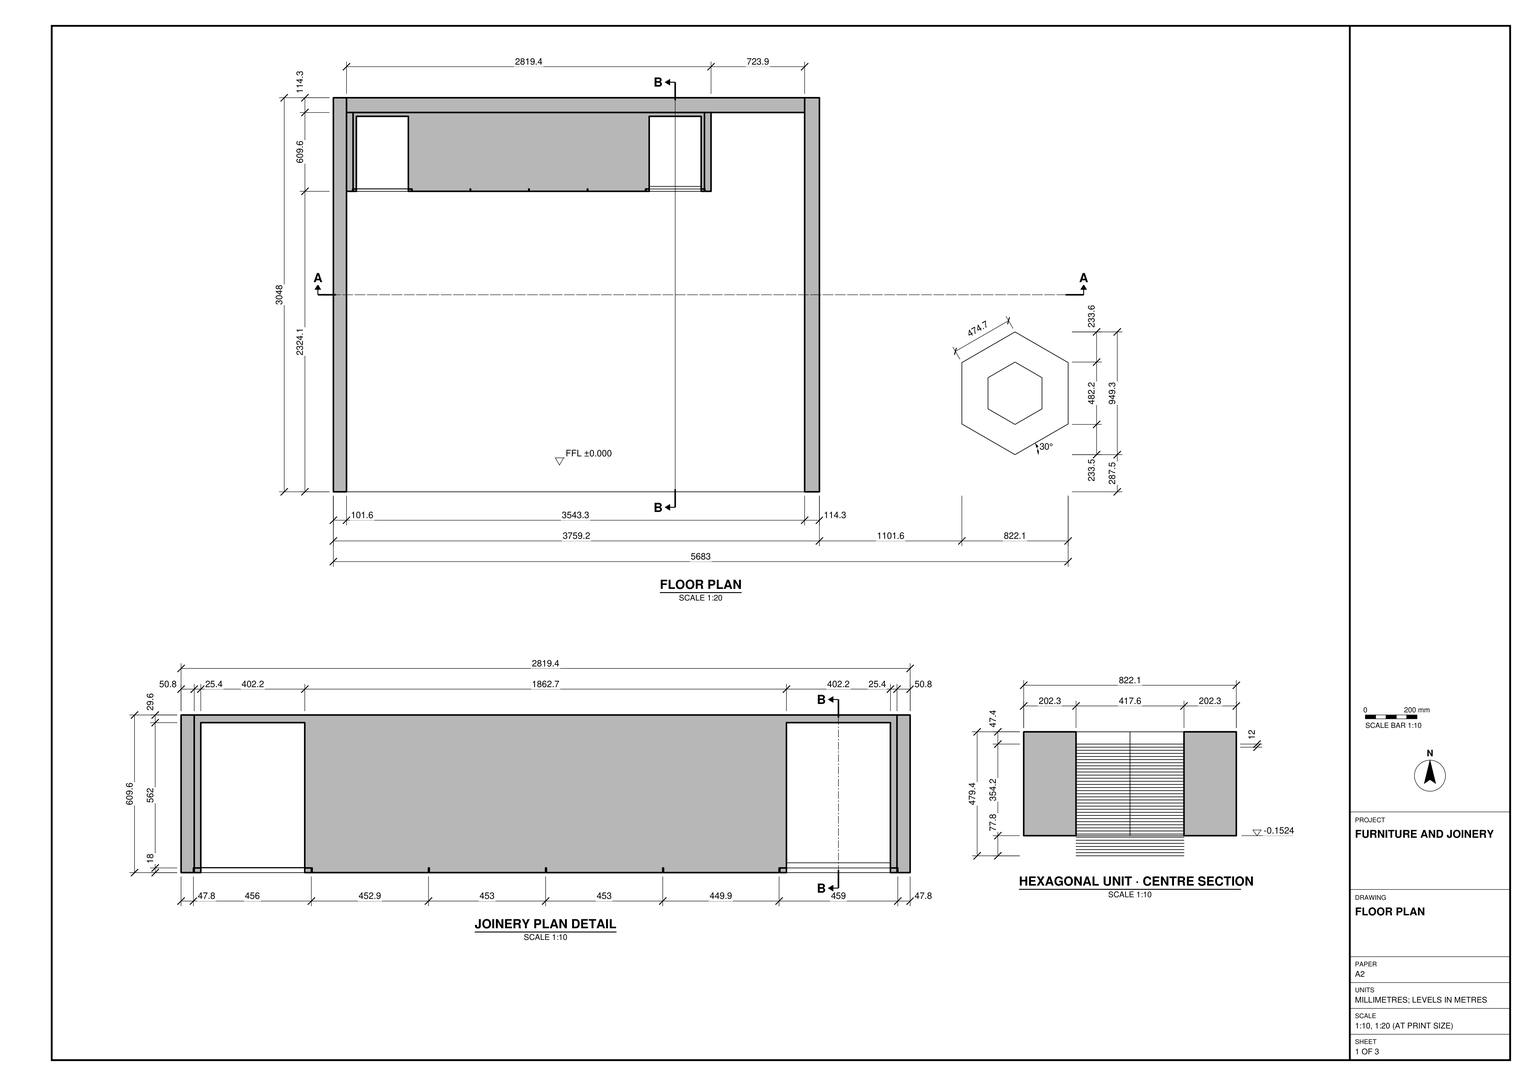
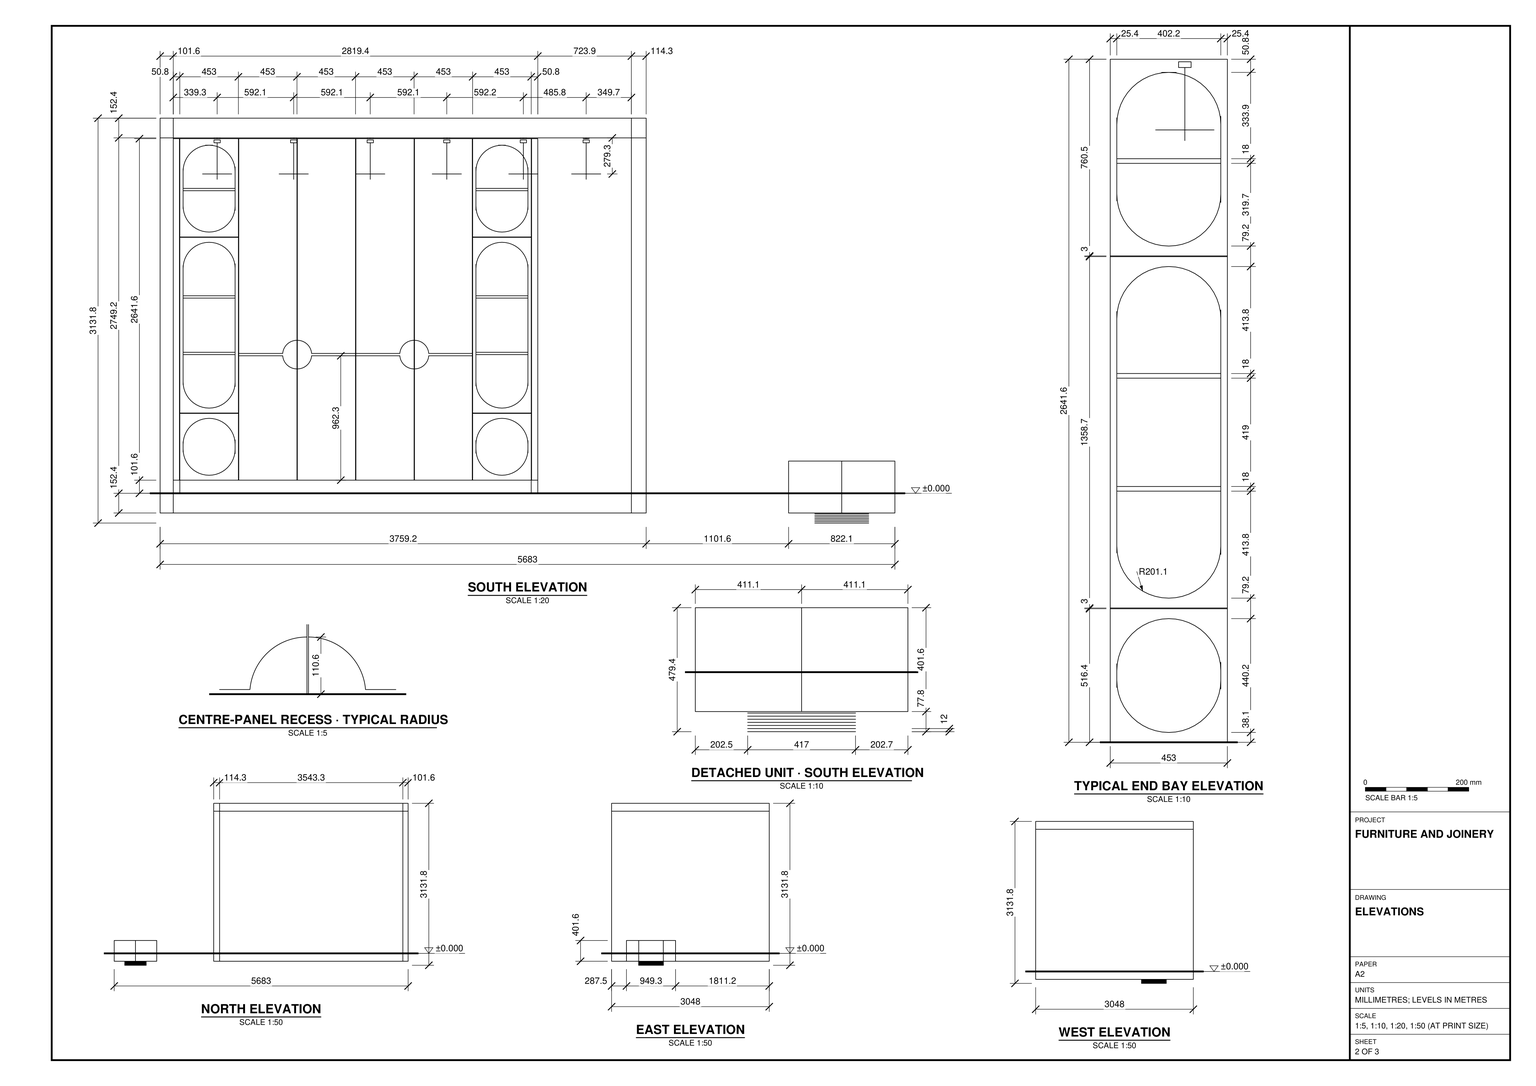
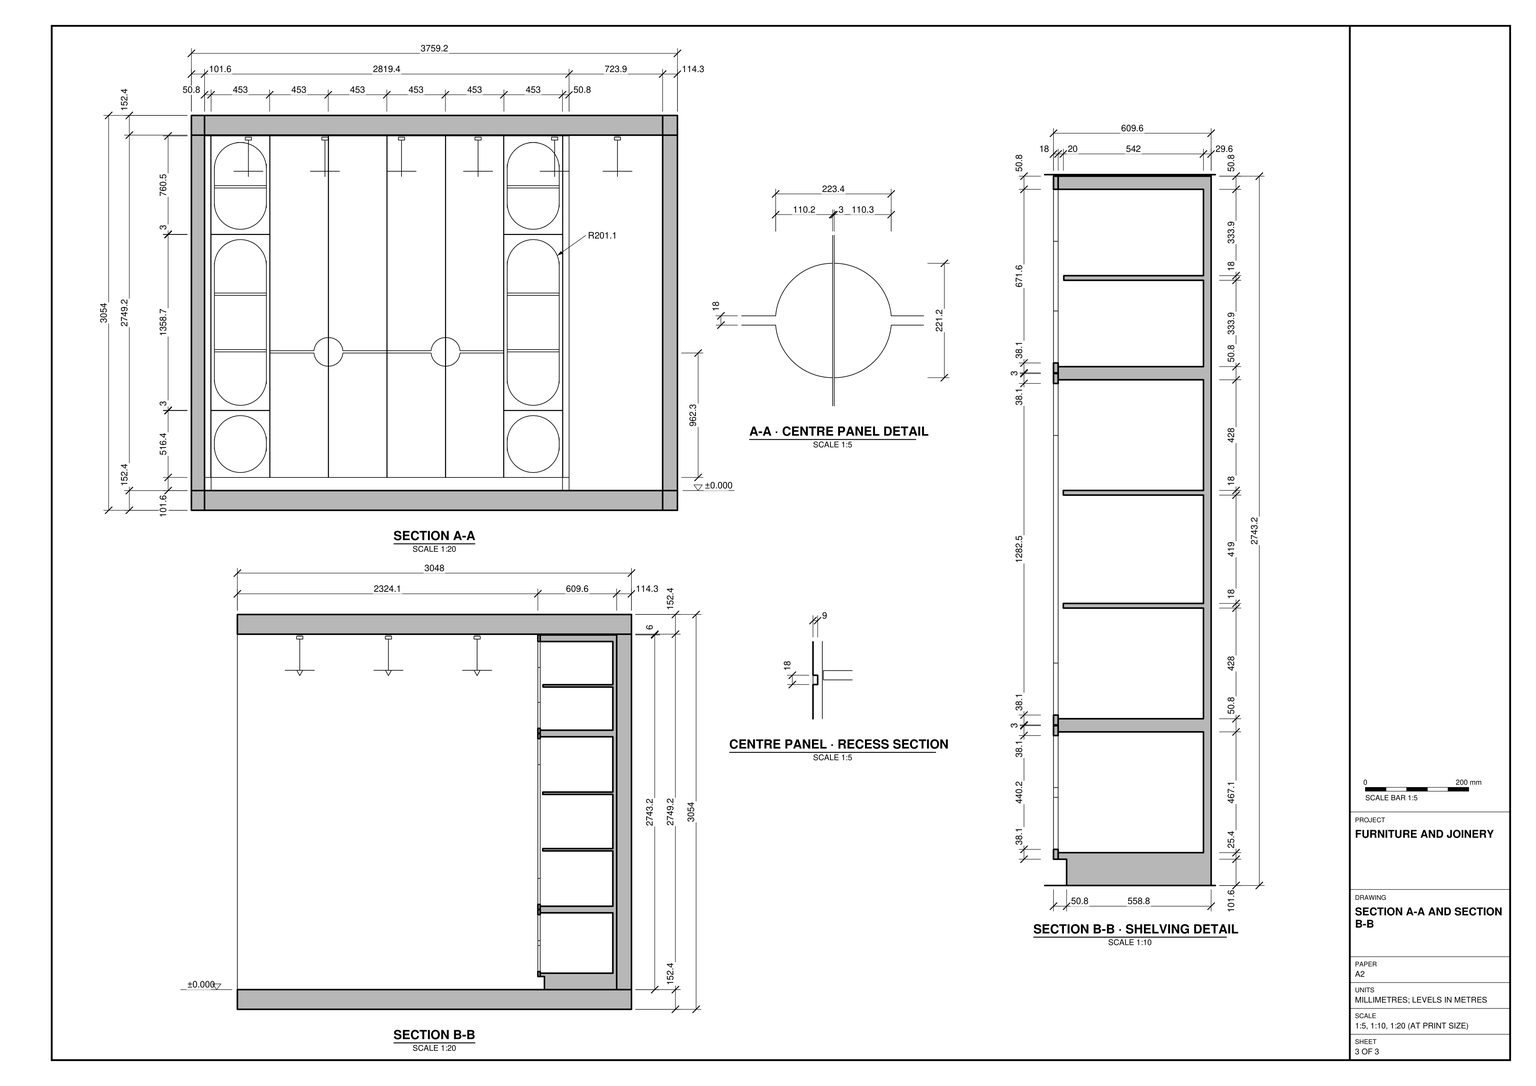
Work in millimetres in SketchUp from task_files/diagram_01.pdf. Model the open-front enclosure, its built-in joinery and the detached hexagonal unit. The complete arrangement spans 5683 mm along X, 3048 mm along Y and 3054 mm along Z. Use the single finished floor level of 0 mm as the datum.

Build the floor slab, side walls, rear wall and overhead slab as shown in plan and section. Viewed from the open front, the left wall is 101.6 mm thick and the right and rear walls are 114.3 mm thick. Set the built-in unit against the rear wall, starting at the left wall and leaving the clear space shown on the right. Model the recessed plinth and the six equal-width bays above it. The four central panels form two pairs; a narrow horizontal recess widens into a circle at the joint of each pair. At either end, form the stacked round-ended openings as openings into shelving, not outlines on a flat face.

Position the detached unit to the right of the enclosure, using the plan for its orientation and the centre section for its underside. Place the ceiling lights as shown. Decor and loose items may be any suitable library components. Keep shell elements and each joinery or furniture piece in separate groups or components, and use components for repeated parts. Save one SketchUp model as output_files/built_in_shelving_enclosure_and_detached_hexagonal_unit.skp.

# SketchUp Ruby script. Lengths in millimetres.
U = 1.mm
M = Sketchup.active_model
def pt(a) = Geom::Point3d.new(a.map { |v| v * U })
def face(e, loops, mat)
  f = e.add_face(loops[0].map { |a| pt(a) })
  loops[1..].each { |l| e.add_face(l.map { |a| pt(a) }).erase! }
  f.material = f.back_material = mat if mat
  f
end
# faces: each face lists its corners as indices into pts; further lists are holes
def faces(e, pts, list, mat = nil) = list.each { |f| face(e, (f[0].is_a?(Array) ? f : [f]).map { |l| l.map { |i| pts[i] } }, mat) }
# xy, xz, yz: faces in a plane at the given z, y or x. An outline is a flat list of corners, or four numbers for a rectangle; further outlines are holes
def ring(l) = l.size == 4 ? [[l[0], l[1]], [l[2], l[1]], [l[2], l[3]], [l[0], l[3]]] : l.each_slice(2).to_a
def flat(e, list, mat, &to3) = list.each { |f| face(e, (f[0].is_a?(Array) ? f : [f]).map { |l| ring(l).map { |u, v| to3.(u, v) } }, mat) }
def xy(e, z, list, mat = nil) = flat(e, list, mat) { |x, y| [x, y, z] }
def xz(e, y, list, mat = nil) = flat(e, list, mat) { |x, z| [x, y, z] }
def yz(e, x, list, mat = nil) = flat(e, list, mat) { |y, z| [x, y, z] }
def lines(e, pts, list) = list.each { |a, b| e.add_line(pt(pts[a]), pt(pts[b])) }
# prism: a flat outline (further loops are holes) pulled along v
def prism(e, loops, v, mat = nil)
  f = face(e, loops, mat); d = Geom::Vector3d.new(v.map { |x| x * U })
  f.pushpull(f.normal.samedirection?(d) ? d.length : -d.length)
end
def box(e, o, s, mat = nil) = prism(e, [[o, [o[0] + s[0], o[1], o[2]], [o[0] + s[0], o[1] + s[1], o[2]], [o[0], o[1] + s[1], o[2]]]], [0, 0, s[2]], mat)
def at(x, y, z, deg = 0) = Geom::Transformation.translation(pt([x, y, z])) * Geom::Transformation.rotation(ORIGIN, Z_AXIS, deg.degrees)
def axes(o, x, y, z) = Geom::Transformation.new([*x, 0, *y, 0, *z, 0, *pt(o).to_a, 1])
def part(name) = M.definitions.add(name)
# library, detail: a bought-in or finely detailed component or shape, given as its bounding box
def library(name, o, s) = part(name).tap { |d| box(d.entities, o, s) }
def detail(e, o, s) = box(e.add_group.entities, o, s)
def put(e, d, t, mat = nil) = e.add_instance(d, t).tap { |i| i.material = mat if mat }
def group(e, t, mat = nil) = e.add_group.tap { |g| g.transformation = t; g.material = mat if mat }.entities
root = M.entities
M.materials.add("Olon-Fresh-Linen-VT10-1K").color = [226, 220, 209]
c1 = part("Group\#1")
xy(c1.entities,0,[[12.7,0,114.3,3048],[114.3,0,3657.6,3048],[3657.6,0,3771.9,3048]])
xy(c1.entities,152.4,[[12.7,0,114.3,3048],[114.3,0,3657.6,3048],[3657.6,0,3771.9,3048]])
xz(c1.entities,0,[[12.7,0,114.3,152.4],[114.3,0,3657.6,152.4],[3657.6,0,3771.9,152.4]])
xz(c1.entities,3048,[[12.7,0,114.3,152.4],[114.3,0,3657.6,152.4],[3657.6,0,3771.9,152.4]])
yz(c1.entities,12.7,[[0,0,3048,152.4]])
yz(c1.entities,114.3,[[0,0,3048,152.4]])
yz(c1.entities,3657.6,[[0,0,3048,152.4]])
yz(c1.entities,3771.9,[[0,0,3048,152.4]])
c2 = library("Group\#2",[0,0,0],[2819.4,609.6,2743.2])
c3 = library("Group\#10",[0,0,0],[226.1,226.1,320.6])
xy(root,0,[[[5271.9,287.5,4860.8,524.8,4860.8,999.5,5271.9,1236.8,5683,999.5,5683,524.8],[5271.9,521,5480.7,641.6,5480.7,882.7,5271.9,1003.2,5063.1,882.7,5063.1,641.6]]])
xy(root,401.6,[[[5271.9,287.5,5683,524.8,5683,999.5,5271.9,1236.8,4860.8,999.5,4860.8,524.8],[5271.9,521,5063.1,641.6,5063.1,882.7,5271.9,1003.2,5480.7,882.7,5480.7,641.6]]])
yz(root,4860.8,[[524.8,0,999.5,401.6]])
yz(root,5063.1,[[641.6,0,882.7,6.2],[641.6,6.2,882.7,18.2],[641.6,18.2,882.7,30.2],[641.6,30.2,882.7,42.2],[641.6,42.2,882.7,54.2],
  [641.6,54.2,882.7,66.2],[641.6,66.2,882.7,78.2],[641.6,78.2,882.7,90.2],[641.6,90.2,882.7,102.2],[641.6,102.2,882.7,114.2],
  [641.6,114.2,882.7,126.2],[641.6,126.2,882.7,138.2],[641.6,138.2,882.7,150.2],[641.6,150.2,882.7,162.2],[641.6,162.2,882.7,174.2],
  [641.6,174.2,882.7,186.2],[641.6,186.2,882.7,198.2],[641.6,198.2,882.7,210.2],[641.6,210.2,882.7,222.2],[641.6,222.2,882.7,234.2],
  [641.6,234.2,882.7,246.2],[641.6,246.2,882.7,258.2],[641.6,258.2,882.7,270.2],[641.6,270.2,882.7,282.2],[641.6,282.2,882.7,294.2],
  [641.6,294.2,882.7,306.2],[641.6,306.2,882.7,318.2],[641.6,318.2,882.7,330.2],[641.6,330.2,882.7,342.2],[641.6,342.2,882.7,354.2],
  [641.6,354.2,882.7,401.6]])
yz(root,5480.7,[[641.6,0,882.7,6.2],[641.6,6.2,882.7,18.2],[641.6,18.2,882.7,30.2],[641.6,30.2,882.7,42.2],[641.6,42.2,882.7,54.2],
  [641.6,54.2,882.7,66.2],[641.6,66.2,882.7,78.2],[641.6,78.2,882.7,90.2],[641.6,90.2,882.7,102.2],[641.6,102.2,882.7,114.2],
  [641.6,114.2,882.7,126.2],[641.6,126.2,882.7,138.2],[641.6,138.2,882.7,150.2],[641.6,150.2,882.7,162.2],[641.6,162.2,882.7,174.2],
  [641.6,174.2,882.7,186.2],[641.6,186.2,882.7,198.2],[641.6,198.2,882.7,210.2],[641.6,210.2,882.7,222.2],[641.6,222.2,882.7,234.2],
  [641.6,234.2,882.7,246.2],[641.6,246.2,882.7,258.2],[641.6,258.2,882.7,270.2],[641.6,270.2,882.7,282.2],[641.6,282.2,882.7,294.2],
  [641.6,294.2,882.7,306.2],[641.6,306.2,882.7,318.2],[641.6,318.2,882.7,330.2],[641.6,330.2,882.7,342.2],[641.6,342.2,882.7,354.2],
  [641.6,354.2,882.7,401.6]])
yz(root,5683,[[524.8,0,999.5,401.6]])
# 42 loose lines left out
p = [[4860.8,524.8,0],[5271.9,287.5,0],[5271.9,287.5,401.6],[4860.8,524.8,401.6],[5683,524.8,0],[5683,524.8,401.6],
  [5063.1,641.6,0],[5063.1,641.6,6.2],[5271.9,521,6.2],[5271.9,521,0],[5480.7,641.6,6.2],[5480.7,641.6,0],
  [5271.9,1003.2,0],[5271.9,1003.2,6.2],[5063.1,882.7,6.2],[5063.1,882.7,0],[5480.7,882.7,0],[5480.7,882.7,6.2],
  [5271.9,1236.8,0],[4860.8,999.5,0],[4860.8,999.5,401.6],[5271.9,1236.8,401.6],[5683,999.5,0],[5683,999.5,401.6],
  [5271.9,521,18.2],[5063.1,641.6,18.2],[5480.7,641.6,18.2],[5063.1,882.7,18.2],[5271.9,1003.2,18.2],[5480.7,882.7,18.2],
  [5271.9,521,30.2],[5063.1,641.6,30.2],[5480.7,641.6,30.2],[5063.1,882.7,30.2],[5271.9,1003.2,30.2],[5480.7,882.7,30.2],
  [5271.9,521,42.2],[5063.1,641.6,42.2],[5480.7,641.6,42.2],[5063.1,882.7,42.2],[5271.9,1003.2,42.2],[5480.7,882.7,42.2],
  [5271.9,521,54.2],[5063.1,641.6,54.2],[5480.7,641.6,54.2],[5063.1,882.7,54.2],[5271.9,1003.2,54.2],[5480.7,882.7,54.2],
  [5271.9,521,66.2],[5063.1,641.6,66.2],[5480.7,641.6,66.2],[5063.1,882.7,66.2],[5271.9,1003.2,66.2],[5480.7,882.7,66.2],
  [5271.9,521,78.2],[5063.1,641.6,78.2],[5480.7,641.6,78.2],[5063.1,882.7,78.2],[5271.9,1003.2,78.2],[5480.7,882.7,78.2],
  [5271.9,521,90.2],[5063.1,641.6,90.2],[5480.7,641.6,90.2],[5063.1,882.7,90.2],[5271.9,1003.2,90.2],[5480.7,882.7,90.2],
  [5271.9,521,102.2],[5063.1,641.6,102.2],[5480.7,641.6,102.2],[5063.1,882.7,102.2],[5271.9,1003.2,102.2],[5480.7,882.7,102.2],
  [5271.9,521,114.2],[5063.1,641.6,114.2],[5480.7,641.6,114.2],[5063.1,882.7,114.2],[5271.9,1003.2,114.2],[5480.7,882.7,114.2],
  [5271.9,521,126.2],[5063.1,641.6,126.2],[5480.7,641.6,126.2],[5063.1,882.7,126.2],[5271.9,1003.2,126.2],[5480.7,882.7,126.2],
  [5271.9,521,138.2],[5063.1,641.6,138.2],[5480.7,641.6,138.2],[5063.1,882.7,138.2],[5271.9,1003.2,138.2],[5480.7,882.7,138.2],
  [5271.9,521,150.2],[5063.1,641.6,150.2],[5480.7,641.6,150.2],[5063.1,882.7,150.2],[5271.9,1003.2,150.2],[5480.7,882.7,150.2],
  [5271.9,521,162.2],[5063.1,641.6,162.2],[5480.7,641.6,162.2],[5063.1,882.7,162.2],[5271.9,1003.2,162.2],[5480.7,882.7,162.2],
  [5271.9,521,174.2],[5063.1,641.6,174.2],[5480.7,641.6,174.2],[5063.1,882.7,174.2],[5271.9,1003.2,174.2],[5480.7,882.7,174.2],
  [5271.9,521,186.2],[5063.1,641.6,186.2],[5480.7,641.6,186.2],[5063.1,882.7,186.2],[5271.9,1003.2,186.2],[5480.7,882.7,186.2],
  [5271.9,521,198.2],[5063.1,641.6,198.2],[5480.7,641.6,198.2],[5063.1,882.7,198.2],[5271.9,1003.2,198.2],[5480.7,882.7,198.2],
  [5271.9,521,210.2],[5063.1,641.6,210.2],[5480.7,641.6,210.2],[5063.1,882.7,210.2],[5271.9,1003.2,210.2],[5480.7,882.7,210.2],
  [5271.9,521,222.2],[5063.1,641.6,222.2],[5480.7,641.6,222.2],[5063.1,882.7,222.2],[5271.9,1003.2,222.2],[5480.7,882.7,222.2],
  [5271.9,521,234.2],[5063.1,641.6,234.2],[5480.7,641.6,234.2],[5063.1,882.7,234.2],[5271.9,1003.2,234.2],[5480.7,882.7,234.2],
  [5271.9,521,246.2],[5063.1,641.6,246.2],[5480.7,641.6,246.2],[5063.1,882.7,246.2],[5271.9,1003.2,246.2],[5480.7,882.7,246.2],
  [5271.9,521,258.2],[5063.1,641.6,258.2],[5480.7,641.6,258.2],[5063.1,882.7,258.2],[5271.9,1003.2,258.2],[5480.7,882.7,258.2],
  [5271.9,521,270.2],[5063.1,641.6,270.2],[5480.7,641.6,270.2],[5063.1,882.7,270.2],[5271.9,1003.2,270.2],[5480.7,882.7,270.2],
  [5271.9,521,282.2],[5063.1,641.6,282.2],[5480.7,641.6,282.2],[5063.1,882.7,282.2],[5271.9,1003.2,282.2],[5480.7,882.7,282.2],
  [5271.9,521,294.2],[5063.1,641.6,294.2],[5480.7,641.6,294.2],[5063.1,882.7,294.2],[5271.9,1003.2,294.2],[5480.7,882.7,294.2],
  [5271.9,521,306.2],[5063.1,641.6,306.2],[5480.7,641.6,306.2],[5063.1,882.7,306.2],[5271.9,1003.2,306.2],[5480.7,882.7,306.2],
  [5271.9,521,318.2],[5063.1,641.6,318.2],[5480.7,641.6,318.2],[5063.1,882.7,318.2],[5271.9,1003.2,318.2],[5480.7,882.7,318.2],
  [5271.9,521,330.2],[5063.1,641.6,330.2],[5480.7,641.6,330.2],[5063.1,882.7,330.2],[5271.9,1003.2,330.2],[5480.7,882.7,330.2],
  [5271.9,521,342.2],[5063.1,641.6,342.2],[5480.7,641.6,342.2],[5063.1,882.7,342.2],[5271.9,1003.2,342.2],[5480.7,882.7,342.2],
  [5271.9,521,354.2],[5063.1,641.6,354.2],[5480.7,641.6,354.2],[5063.1,882.7,354.2],[5271.9,1003.2,354.2],[5480.7,882.7,354.2],
  [5271.9,521,401.6],[5063.1,641.6,401.6],[5480.7,641.6,401.6],[5063.1,882.7,401.6],[5271.9,1003.2,401.6],[5480.7,882.7,401.6]]
faces(root,p,[[0,1,2,3],[1,4,5,2],[6,7,8,9],[9,8,10,11],[12,13,14,15],[16,17,13,12],[18,19,20,21],[22,18,21,23],
  [24,8,7,25],[26,10,8,24],[27,14,13,28],[28,13,17,29],[30,24,25,31],[32,26,24,30],[33,27,28,34],[34,28,29,35],
  [36,30,31,37],[38,32,30,36],[39,33,34,40],[40,34,35,41],[42,36,37,43],[44,38,36,42],[45,39,40,46],[46,40,41,47],
  [48,42,43,49],[50,44,42,48],[51,45,46,52],[52,46,47,53],[54,48,49,55],[56,50,48,54],[57,51,52,58],[58,52,53,59],
  [60,54,55,61],[62,56,54,60],[63,57,58,64],[64,58,59,65],[66,60,61,67],[68,62,60,66],[69,63,64,70],[70,64,65,71],
  [72,66,67,73],[74,68,66,72],[75,69,70,76],[76,70,71,77],[78,72,73,79],[80,74,72,78],[81,75,76,82],[82,76,77,83],
  [84,78,79,85],[86,80,78,84],[87,81,82,88],[88,82,83,89],[90,84,85,91],[92,86,84,90],[93,87,88,94],[94,88,89,95],
  [96,90,91,97],[98,92,90,96],[99,93,94,100],[100,94,95,101],[102,96,97,103],[104,98,96,102],[105,99,100,106],[106,100,101,107],
  [108,102,103,109],[110,104,102,108],[111,105,106,112],[112,106,107,113],[114,108,109,115],[116,110,108,114],[117,111,112,118],[118,112,113,119],
  [120,114,115,121],[122,116,114,120],[123,117,118,124],[124,118,119,125],[126,120,121,127],[128,122,120,126],[129,123,124,130],[130,124,125,131],
  [132,126,127,133],[134,128,126,132],[135,129,130,136],[136,130,131,137],[138,132,133,139],[140,134,132,138],[141,135,136,142],[142,136,137,143],
  [144,138,139,145],[146,140,138,144],[147,141,142,148],[148,142,143,149],[150,144,145,151],[152,146,144,150],[153,147,148,154],[154,148,149,155],
  [156,150,151,157],[158,152,150,156],[159,153,154,160],[160,154,155,161],[162,156,157,163],[164,158,156,162],[165,159,160,166],[166,160,161,167],
  [168,162,163,169],[170,164,162,168],[171,165,166,172],[172,166,167,173],[174,168,169,175],[176,170,168,174],[177,171,172,178],[178,172,173,179],
  [180,174,175,181],[182,176,174,180],[183,177,178,184],[184,178,179,185],[186,180,181,187],[188,182,180,186],[189,183,184,190],[190,184,185,191],
  [192,186,187,193],[194,188,186,192],[195,189,190,196],[196,190,191,197],[198,192,193,199],[200,194,192,198],[201,195,196,202],[202,196,197,203]])
put(root,c1,at(-12.7,0,0))
g1 = group(root,at(-12.7,2933.7,152.4))
box(g1,[114.3,0,0],[3543.3,114.3,2749.2])
put(root,c2,at(101.6,2324.1,152.4),"Olon-Fresh-Linen-VT10-1K")
g2 = group(root,at(152.4,2324.1,254),"Olon-Fresh-Linen-VT10-1K")
prism(g2,[[[0,18,516.4],[453,18,516.4],[453,18,0],[0,18,0]],[[25.4,18,277.2],[25.4,18,239.2],[27.1,18,212.9],[32.3,18,187.1],[40.7,18,162.2],[52.3,18,138.6],[67,18,116.8],[84.3,18,97],[104.1,18,79.7],[125.9,18,65],[149.5,18,53.4],[174.4,18,45],[200.2,18,39.8],[226.5,18,38.1],[252.7,18,39.8],[278.5,18,45],[303.4,18,53.4],[327,18,65],[348.9,18,79.7],[368.7,18,97],[386,18,116.8],[400.6,18,138.6],[412.3,18,162.2],[420.7,18,187.1],[425.8,18,212.9],[427.6,18,239.2],[427.6,18,277.2],[425.8,18,303.5],[420.7,18,329.3],[412.3,18,354.2],[400.6,18,377.8],[386,18,399.6],[368.7,18,419.4],[348.9,18,436.7],[327,18,451.4],[303.4,18,463],[278.5,18,471.4],[252.7,18,476.6],[226.5,18,478.3],[200.2,18,476.6],[174.4,18,471.4],[149.5,18,463],[125.9,18,451.4],[104.1,18,436.7],[84.3,18,419.4],[67,18,399.6],[52.3,18,377.8],[40.7,18,354.2],[32.3,18,329.3],[27.1,18,303.5]]],[0,-18,0])
g3 = group(root,at(2417.2,2324.1,254),"Olon-Fresh-Linen-VT10-1K")
prism(g3,[[[0,18,516.4],[453,18,516.4],[453,18,0],[0,18,0]],[[25.4,18,277.2],[25.4,18,239.2],[27.1,18,212.9],[32.3,18,187.1],[40.7,18,162.2],[52.3,18,138.6],[67,18,116.8],[84.3,18,97],[104.1,18,79.7],[125.9,18,65],[149.5,18,53.4],[174.4,18,45],[200.2,18,39.8],[226.5,18,38.1],[252.7,18,39.8],[278.5,18,45],[303.4,18,53.4],[327,18,65],[348.9,18,79.7],[368.7,18,97],[386,18,116.8],[400.6,18,138.6],[412.3,18,162.2],[420.7,18,187.1],[425.8,18,212.9],[427.6,18,239.2],[427.6,18,277.2],[425.8,18,303.5],[420.7,18,329.3],[412.3,18,354.2],[400.6,18,377.8],[386,18,399.6],[368.7,18,419.4],[348.9,18,436.7],[327,18,451.4],[303.4,18,463],[278.5,18,471.4],[252.7,18,476.6],[226.5,18,478.3],[200.2,18,476.6],[174.4,18,471.4],[149.5,18,463],[125.9,18,451.4],[104.1,18,436.7],[84.3,18,419.4],[67,18,399.6],[52.3,18,377.8],[40.7,18,354.2],[32.3,18,329.3],[27.1,18,303.5]]],[0,-18,0])
g4 = group(root,at(0,0,152.4))
box(g4,[0,0,0],[101.6,3048,2749.2])
g5 = group(root,at(3644.9,0,152.4))
box(g5,[0,0,0],[114.3,3048,2749.2])
put(root,c1,at(-12.7,0,2901.6))
put(root,c3,at(327.9,1741.2,2581))
put(root,c3,at(920,1741.2,2581))
put(root,c3,at(1512.1,1741.2,2581))
put(root,c3,at(2104.3,1741.2,2581))
put(root,c3,at(2696.4,1741.2,2581))
put(root,c3,at(3182.2,1741.2,2581))
put(root,c3,at(3182.2,1055.4,2581))
put(root,c3,at(1512.1,1055.4,2581))
put(root,c3,at(2104.3,1055.4,2581))
put(root,c3,at(2696.4,1055.4,2581))
put(root,c3,at(920,1055.4,2581))
put(root,c3,at(327.9,1055.4,2581))
put(root,c3,at(3182.2,369.6,2581))
put(root,c3,at(1512.1,369.6,2581))
put(root,c3,at(2104.3,369.6,2581))
put(root,c3,at(2696.4,369.6,2581))
put(root,c3,at(920,369.6,2581))
put(root,c3,at(327.9,369.6,2581))
